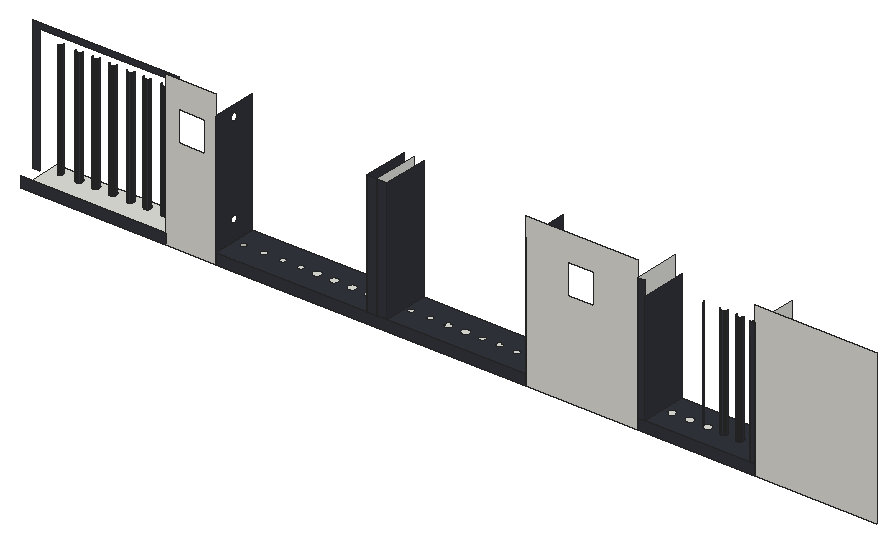
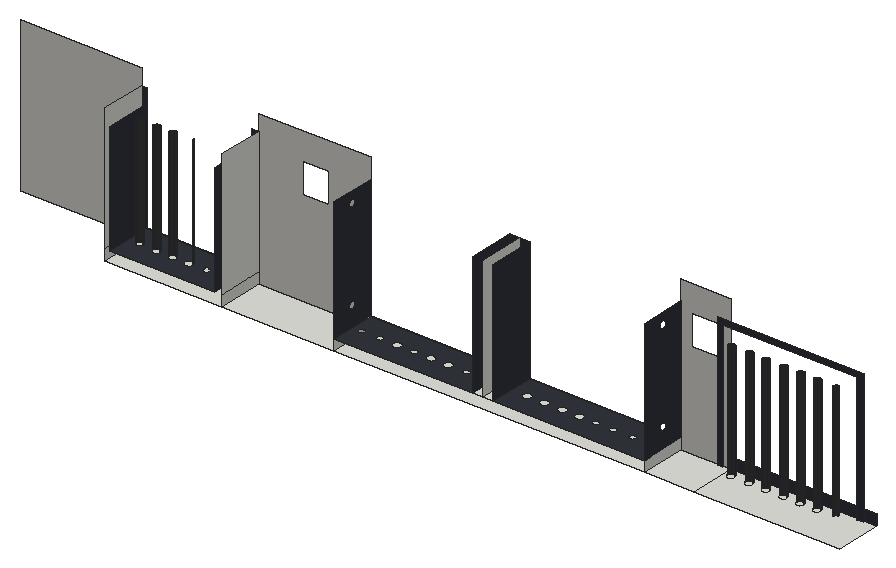
# SketchUp Ruby script. Lengths in inches.
U = 1.inch
M = Sketchup.active_model
def pt(a) = Geom::Point3d.new(a.map { |v| v * U })
def face(e, loops, mat)
  f = e.add_face(loops[0].map { |a| pt(a) })
  loops[1..].each { |l| e.add_face(l.map { |a| pt(a) }).erase! }
  f.material = f.back_material = mat if mat
  f
end
# faces: each face lists its corners as indices into pts; further lists are holes
def faces(e, pts, list, mat = nil) = list.each { |f| face(e, (f[0].is_a?(Array) ? f : [f]).map { |l| l.map { |i| pts[i] } }, mat) }
# xy, xz, yz: faces in a plane at the given z, y or x. An outline is a flat list of corners, or four numbers for a rectangle; further outlines are holes
def ring(l) = l.size == 4 ? [[l[0], l[1]], [l[2], l[1]], [l[2], l[3]], [l[0], l[3]]] : l.each_slice(2).to_a
def flat(e, list, mat, &to3) = list.each { |f| face(e, (f[0].is_a?(Array) ? f : [f]).map { |l| ring(l).map { |u, v| to3.(u, v) } }, mat) }
def xy(e, z, list, mat = nil) = flat(e, list, mat) { |x, y| [x, y, z] }
def xz(e, y, list, mat = nil) = flat(e, list, mat) { |x, z| [x, y, z] }
def yz(e, x, list, mat = nil) = flat(e, list, mat) { |y, z| [x, y, z] }
def lines(e, pts, list) = list.each { |a, b| e.add_line(pt(pts[a]), pt(pts[b])) }
# prism: a flat outline (further loops are holes) pulled along v
def prism(e, loops, v, mat = nil)
  f = face(e, loops, mat); d = Geom::Vector3d.new(v.map { |x| x * U })
  f.pushpull(f.normal.samedirection?(d) ? d.length : -d.length)
end
def box(e, o, s, mat = nil) = prism(e, [[o, [o[0] + s[0], o[1], o[2]], [o[0] + s[0], o[1] + s[1], o[2]], [o[0], o[1] + s[1], o[2]]]], [0, 0, s[2]], mat)
def at(x, y, z, deg = 0) = Geom::Transformation.translation(pt([x, y, z])) * Geom::Transformation.rotation(ORIGIN, Z_AXIS, deg.degrees)
def axes(o, x, y, z) = Geom::Transformation.new([*x, 0, *y, 0, *z, 0, *pt(o).to_a, 1])
def part(name) = M.definitions.add(name)
# library, detail: a bought-in or finely detailed component or shape, given as its bounding box
def library(name, o, s) = part(name).tap { |d| box(d.entities, o, s) }
def detail(e, o, s) = box(e.add_group.entities, o, s)
def put(e, d, t, mat = nil) = e.add_instance(d, t).tap { |i| i.material = mat if mat }
def group(e, t, mat = nil) = e.add_group.tap { |g| g.transformation = t; g.material = mat if mat }.entities
root = M.entities
M.materials.add("[Formica Laminate Dark]1").color = [50, 53, 60]
M.materials.add("[Terrazzo Tile Light]").color = [219, 217, 210]
xy(root,0,[[1357.59,0,1765.91,129.42],[1765.91,0,1905.75,129.42],[1905.75,0,2778.47,129.42],[2778.47,0,3092.67,129.42],[3092.67,0,3421.78,129.42]])
xy(root,29.875,[[2330.84,0,2358.7,129.42],[2358.7,0,2386.55,129.42],[1472.87,55.58,1470.36,55.72,1467.97,56.51,1465.87,57.89,1464.2,59.76,1463.07,62.01,1462.56,64.47,1462.7,66.98,1463.49,69.36,1464.86,71.46,1466.74,73.14,1468.98,74.27,1471.44,74.78,1473.95,74.64,1476.34,73.85,1478.4375,72.47,1480.11,70.6,1481.24,68.35,1481.75,65.89,1481.61,63.38,1480.82,61,1479.45,58.9,1477.57,57.22,1475.33,56.09],[1518.99,55.58,1516.48,55.72,1514.1,56.51,1512,57.89,1510.32,59.76,1509.19,62.01,1508.68,64.47,1508.82,66.98,1509.61,69.36,1510.99,71.46,1512.86,73.14,1515.11,74.27,1517.57,74.78,1520.08,74.64,1522.46,73.85,1524.5625,72.47,1526.24,70.6,1527.37,68.35,1527.88,65.89,1527.74,63.38,1526.95,61,1525.57,58.9,1523.7,57.22,1521.45,56.09],[1566.87,55.58,1564.36,55.72,1561.97,56.51,1559.87,57.89,1558.2,59.76,1557.07,62.01,1556.56,64.47,1556.7,66.98,1557.49,69.36,1558.86,71.46,1560.74,73.14,1562.98,74.27,1565.44,74.78,1567.95,74.64,1570.34,73.85,1572.4375,72.47,1574.11,70.6,1575.24,68.35,1575.75,65.89,1575.61,63.38,1574.82,61,1573.45,58.9,1571.57,57.22,1569.33,56.09],
  [1616.43,55.58,1613.92,55.72,1611.54,56.51,1609.43,57.89,1607.76,59.76,1606.63,62.01,1606.12,64.47,1606.26,66.98,1607.05,69.36,1608.43,71.46,1610.3,73.14,1612.54,74.27,1615,74.78,1617.51,74.64,1619.9,73.85,1622,72.47,1623.67,70.6,1624.8,68.35,1625.32,65.89,1625.17,63.38,1624.39,61,1623.01,58.9,1621.13,57.22,1618.89,56.09],[1663.87,55.58,1661.36,55.72,1658.97,56.51,1656.87,57.89,1655.2,59.76,1654.07,62.01,1653.56,64.47,1653.7,66.98,1654.49,69.36,1655.86,71.46,1657.74,73.14,1659.98,74.27,1662.44,74.78,1664.95,74.64,1667.34,73.85,1669.4375,72.47,1671.11,70.6,1672.24,68.35,1672.75,65.89,1672.61,63.38,1671.82,61,1670.45,58.9,1668.57,57.22,1666.33,56.09],[1714.37,55.58,1711.86,55.72,1709.47,56.51,1707.37,57.89,1705.7,59.76,1704.57,62.01,1704.06,64.47,1704.2,66.98,1704.99,69.36,1706.36,71.46,1708.24,73.14,1710.48,74.27,1712.94,74.78,1715.45,74.64,1717.84,73.85,1719.9375,72.47,1721.61,70.6,1722.74,68.35,1723.25,65.89,1723.11,63.38,1722.32,61,1720.95,58.9,1719.07,57.22,1716.83,56.09],[2139.99,55.58,2137.48,55.72,2135.1,56.51,2133,57.89,2131.32,59.76,2130.19,62.01,2129.68,64.47,2129.82,66.98,2130.61,69.36,2131.99,71.46,2133.86,73.14,2136.11,74.27,2138.57,74.78,2141.08,74.64,2143.46,73.85,2145.5625,72.47,2147.24,70.6,2148.37,68.35,2148.88,65.89,2148.74,63.38,2147.95,61,2146.57,58.9,2144.7,57.22,2142.45,56.09],[2187.99,55.58,2185.48,55.72,2183.1,56.51,2181,57.89,2179.32,59.76,2178.19,62.01,2177.68,64.47,2177.82,66.98,2178.61,69.36,2179.99,71.46,2181.86,73.14,2184.11,74.27,2186.57,74.78,2189.08,74.64,2191.46,73.85,2193.5625,72.47,2195.24,70.6,2196.37,68.35,2196.88,65.89,2196.74,63.38,2195.95,61,2194.57,58.9,2192.7,57.22,2190.45,56.09],
  [2238.68,55.58,2236.17,55.72,2233.79,56.51,2231.68,57.89,2230.01,59.76,2228.88,62.01,2228.37,64.47,2228.51,66.98,2229.3,69.36,2230.68,71.46,2232.55,73.14,2234.79,74.27,2237.25,74.78,2239.76,74.64,2242.15,73.85,2244.25,72.47,2245.92,70.6,2247.05,68.35,2247.57,65.89,2247.42,63.38,2246.64,61,2245.26,58.9,2243.38,57.22,2241.14,56.09],[2286.99,55.58,2284.48,55.72,2282.1,56.51,2280,57.89,2278.32,59.76,2277.19,62.01,2276.68,64.47,2276.82,66.98,2277.61,69.36,2278.99,71.46,2280.86,73.14,2283.11,74.27,2285.57,74.78,2288.08,74.64,2290.46,73.85,2292.5625,72.47,2294.24,70.6,2295.37,68.35,2295.88,65.89,2295.74,63.38,2294.95,61,2293.57,58.9,2291.7,57.22,2289.45,56.09],[2508.93,55.58,2506.42,55.72,2504.04,56.51,2501.93,57.89,2500.26,59.76,2499.13,62.01,2498.62,64.47,2498.76,66.98,2499.55,69.36,2500.93,71.46,2502.8,73.14,2505.04,74.27,2507.5,74.78,2510.01,74.64,2512.4,73.85,2514.5,72.47,2516.17,70.6,2517.3,68.35,2517.82,65.89,2517.67,63.38,2516.89,61,2515.51,58.9,2513.63,57.22,2511.39,56.09],[2557.49,55.58,2554.98,55.72,2552.6,56.51,2550.5,57.89,2548.82,59.76,2547.69,62.01,2547.18,64.47,2547.32,66.98,2548.11,69.36,2549.49,71.46,2551.36,73.14,2553.61,74.27,2556.07,74.78,2558.58,74.64,2560.96,73.85,2563.0625,72.47,2564.74,70.6,2565.87,68.35,2566.38,65.89,2566.24,63.38,2565.45,61,2564.07,58.9,2562.2,57.22,2559.95,56.09],[2651.93,55.58,2649.42,55.72,2647.04,56.51,2644.93,57.89,2643.26,59.76,2642.13,62.01,2641.62,64.47,2641.76,66.98,2642.55,69.36,2643.93,71.46,2645.8,73.14,2648.04,74.27,2650.5,74.78,2653.01,74.64,2655.4,73.85,2657.5,72.47,2659.17,70.6,2660.3,68.35,2660.82,65.89,2660.67,63.38,2659.89,61,2658.51,58.9,2656.63,57.22,2654.39,56.09],
  [3137.87,55.58,3135.36,55.72,3132.97,56.51,3130.87,57.89,3129.2,59.76,3128.07,62.01,3127.56,64.47,3127.7,66.98,3128.49,69.36,3129.86,71.46,3131.74,73.14,3133.98,74.27,3136.44,74.78,3138.95,74.64,3141.34,73.85,3143.4375,72.47,3145.11,70.6,3146.24,68.35,3146.75,65.89,3146.61,63.38,3145.82,61,3144.45,58.9,3142.57,57.22,3140.33,56.09],[3187.99,55.58,3185.48,55.72,3183.1,56.51,3181,57.89,3179.32,59.76,3178.19,62.01,3177.68,64.47,3177.82,66.98,3178.61,69.36,3179.99,71.46,3181.86,73.14,3184.11,74.27,3186.57,74.78,3189.08,74.64,3191.46,73.85,3193.5625,72.47,3195.24,70.6,3196.37,68.35,3196.88,65.89,3196.74,63.38,3195.95,61,3194.57,58.9,3192.7,57.22,3190.45,56.09],[3236.93,55.58,3234.42,55.72,3232.04,56.51,3229.93,57.89,3228.26,59.76,3227.13,62.01,3226.62,64.47,3226.76,66.98,3227.55,69.36,3228.93,71.46,3230.8,73.14,3233.04,74.27,3235.5,74.78,3238.01,74.64,3240.4,73.85,3242.5,72.47,3244.17,70.6,3245.3,68.35,3245.82,65.89,3245.67,63.38,3244.89,61,3243.51,58.9,3241.63,57.22,3239.39,56.09],[3282.55,55.58,3280.05,55.72,3277.66,56.51,3275.56,57.89,3273.89,59.76,3272.76,62.01,3272.24,64.47,3272.39,66.98,3273.17,69.36,3274.55,71.46,3276.43,73.14,3278.67,74.27,3281.13,74.78,3283.64,74.64,3286.02,73.85,3288.125,72.47,3289.8,70.6,3290.93,68.35,3291.44,65.89,3291.3,63.38,3290.51,61,3289.13,58.9,3287.26,57.22,3285.01,56.09],[3328.68,55.58,3326.17,55.72,3323.79,56.51,3321.68,57.89,3320.01,59.76,3318.88,62.01,3318.37,64.47,3318.51,66.98,3319.3,69.36,3320.68,71.46,3322.55,73.14,3324.79,74.27,3327.25,74.78,3329.76,74.64,3332.15,73.85,3334.25,72.47,3335.92,70.6,3337.05,68.35,3337.57,65.89,3337.42,63.38,3336.64,61,3335.26,58.9,3333.38,57.22,3331.14,56.09]])
xy(root,29.875,[[[1905.75,0,2330.84,129.42],[2139.99,55.58,2137.48,55.72,2135.1,56.51,2133,57.89,2131.32,59.76,2130.19,62.01,2129.68,64.47,2129.82,66.98,2130.61,69.36,2131.99,71.46,2133.86,73.14,2136.11,74.27,2138.57,74.78,2141.08,74.64,2143.46,73.85,2145.5625,72.47,2147.24,70.6,2148.37,68.35,2148.88,65.89,2148.74,63.38,2147.95,61,2146.57,58.9,2144.7,57.22,2142.45,56.09],[2187.99,55.58,2185.48,55.72,2183.1,56.51,2181,57.89,2179.32,59.76,2178.19,62.01,2177.68,64.47,2177.82,66.98,2178.61,69.36,2179.99,71.46,2181.86,73.14,2184.11,74.27,2186.57,74.78,2189.08,74.64,2191.46,73.85,2193.5625,72.47,2195.24,70.6,2196.37,68.35,2196.88,65.89,2196.74,63.38,2195.95,61,2194.57,58.9,2192.7,57.22,2190.45,56.09],[2238.68,55.58,2236.17,55.72,2233.79,56.51,2231.68,57.89,2230.01,59.76,2228.88,62.01,2228.37,64.47,2228.51,66.98,2229.3,69.36,2230.68,71.46,2232.55,73.14,2234.79,74.27,2237.25,74.78,2239.76,74.64,2242.15,73.85,2244.25,72.47,2245.92,70.6,2247.05,68.35,2247.57,65.89,2247.42,63.38,2246.64,61,2245.26,58.9,2243.38,57.22,2241.14,56.09],[2286.99,55.58,2284.48,55.72,2282.1,56.51,2280,57.89,2278.32,59.76,2277.19,62.01,2276.68,64.47,2276.82,66.98,2277.61,69.36,2278.99,71.46,2280.86,73.14,2283.11,74.27,2285.57,74.78,2288.08,74.64,2290.46,73.85,2292.5625,72.47,2294.24,70.6,2295.37,68.35,2295.88,65.89,2295.74,63.38,2294.95,61,2293.57,58.9,2291.7,57.22,2289.45,56.09],[2094.55,55.58,2092.05,55.72,2089.66,56.51,2087.56,57.89,2085.89,59.76,2084.76,62.01,2084.24,64.47,2084.39,66.98,2085.17,69.36,2086.55,71.46,2088.43,73.14,2090.67,74.27,2093.13,74.78,2095.64,74.64,2098.02,73.85,2100.125,72.47,2101.8,70.6,2102.93,68.35,2103.44,65.89,2103.3,63.38,2102.51,61,2101.13,58.9,2099.26,57.22,2097.01,56.09],[2044.37,55.58,2041.86,55.72,2039.47,56.51,2037.37,57.89,2035.7,59.76,2034.57,62.01,2034.06,64.47,2034.2,66.98,2034.99,69.36,2036.36,71.46,2038.24,73.14,2040.48,74.27,2042.94,74.78,2045.45,74.64,2047.84,73.85,2049.9375,72.47,2051.61,70.6,2052.74,68.35,2053.25,65.89,2053.11,63.38,2052.32,61,2050.95,58.9,2049.07,57.22,2046.83,56.09],[1934.18,55.58,1931.67,55.72,1929.29,56.51,1927.18,57.89,1925.51,59.76,1924.38,62.01,1923.87,64.47,1924.01,66.98,1924.8,69.36,1926.18,71.46,1928.05,73.14,1930.29,74.27,1932.75,74.78,1935.26,74.64,1937.65,73.85,1939.75,72.47,1941.42,70.6,1942.55,68.35,1943.07,65.89,1942.92,63.38,1942.14,61,1940.76,58.9,1938.88,57.22,1936.64,56.09],[1991.49,55.58,1988.98,55.72,1986.6,56.51,1984.5,57.89,1982.82,59.76,1981.69,62.01,1981.18,64.47,1981.32,66.98,1982.11,69.36,1983.49,71.46,1985.36,73.14,1987.61,74.27,1990.07,74.78,1992.58,74.64,1994.96,73.85,1997.0625,72.47,1998.74,70.6,1999.87,68.35,2000.38,65.89,2000.24,63.38,1999.45,61,1998.07,58.9,1996.2,57.22,1993.95,56.09]],[[2386.55,0,2778.47,129.42],[2508.93,55.58,2506.42,55.72,2504.04,56.51,2501.93,57.89,2500.26,59.76,2499.13,62.01,2498.62,64.47,2498.76,66.98,2499.55,69.36,2500.93,71.46,2502.8,73.14,2505.04,74.27,2507.5,74.78,2510.01,74.64,2512.4,73.85,2514.5,72.47,2516.17,70.6,2517.3,68.35,2517.82,65.89,2517.67,63.38,2516.89,61,2515.51,58.9,2513.63,57.22,2511.39,56.09],[2557.49,55.58,2554.98,55.72,2552.6,56.51,2550.5,57.89,2548.82,59.76,2547.69,62.01,2547.18,64.47,2547.32,66.98,2548.11,69.36,2549.49,71.46,2551.36,73.14,2553.61,74.27,2556.07,74.78,2558.58,74.64,2560.96,73.85,2563.0625,72.47,2564.74,70.6,2565.87,68.35,2566.38,65.89,2566.24,63.38,2565.45,61,2564.07,58.9,2562.2,57.22,2559.95,56.09],[2651.93,55.58,2649.42,55.72,2647.04,56.51,2644.93,57.89,2643.26,59.76,2642.13,62.01,2641.62,64.47,2641.76,66.98,2642.55,69.36,2643.93,71.46,2645.8,73.14,2648.04,74.27,2650.5,74.78,2653.01,74.64,2655.4,73.85,2657.5,72.47,2659.17,70.6,2660.3,68.35,2660.82,65.89,2660.67,63.38,2659.89,61,2658.51,58.9,2656.63,57.22,2654.39,56.09],[2752.12,55.58,2749.61,55.72,2747.22,56.51,2745.12,57.89,2743.45,59.76,2742.32,62.01,2741.81,64.47,2741.95,66.98,2742.74,69.36,2744.11,71.46,2745.99,73.14,2748.23,74.27,2750.69,74.78,2753.2,74.64,2755.59,73.85,2757.6875,72.47,2759.36,70.6,2760.49,68.35,2761,65.89,2760.86,63.38,2760.07,61,2758.7,58.9,2756.82,57.22,2754.58,56.09],[2700.93,55.58,2698.42,55.72,2696.04,56.51,2693.93,57.89,2692.26,59.76,2691.13,62.01,2690.62,64.47,2690.76,66.98,2691.55,69.36,2692.93,71.46,2694.8,73.14,2697.04,74.27,2699.5,74.78,2702.01,74.64,2704.4,73.85,2706.5,72.47,2708.17,70.6,2709.3,68.35,2709.82,65.89,2709.67,63.38,2708.89,61,2707.51,58.9,2705.63,57.22,2703.39,56.09],[2604.55,55.58,2602.05,55.72,2599.66,56.51,2597.56,57.89,2595.89,59.76,2594.76,62.01,2594.24,64.47,2594.39,66.98,2595.17,69.36,2596.55,71.46,2598.43,73.14,2600.67,74.27,2603.13,74.78,2605.64,74.64,2608.02,73.85,2610.125,72.47,2611.8,70.6,2612.93,68.35,2613.44,65.89,2613.3,63.38,2612.51,61,2611.13,58.9,2609.26,57.22,2607.01,56.09],[2458.12,55.58,2455.61,55.72,2453.22,56.51,2451.12,57.89,2449.45,59.76,2448.32,62.01,2447.81,64.47,2447.95,66.98,2448.74,69.36,2450.11,71.46,2451.99,73.14,2454.23,74.27,2456.69,74.78,2459.2,74.64,2461.59,73.85,2463.6875,72.47,2465.36,70.6,2466.49,68.35,2467,65.89,2466.86,63.38,2466.07,61,2464.7,58.9,2462.82,57.22,2460.58,56.09],[2404.12,55.58,2401.61,55.72,2399.22,56.51,2397.12,57.89,2395.45,59.76,2394.32,62.01,2393.81,64.47,2393.95,66.98,2394.74,69.36,2396.11,71.46,2397.99,73.14,2400.23,74.27,2402.69,74.78,2405.2,74.64,2407.59,73.85,2409.6875,72.47,2411.36,70.6,2412.49,68.35,2413,65.89,2412.86,63.38,2412.07,61,2410.7,58.9,2408.82,57.22,2406.58,56.09]],[[3111.49,0,3407.39,129.42],[3328.68,55.58,3326.17,55.72,3323.79,56.51,3321.68,57.89,3320.01,59.76,3318.88,62.01,3318.37,64.47,3318.51,66.98,3319.3,69.36,3320.68,71.46,3322.55,73.14,3324.79,74.27,3327.25,74.78,3329.76,74.64,3332.15,73.85,3334.25,72.47,3335.92,70.6,3337.05,68.35,3337.57,65.89,3337.42,63.38,3336.64,61,3335.26,58.9,3333.38,57.22,3331.14,56.09],[3137.87,55.58,3135.36,55.72,3132.97,56.51,3130.87,57.89,3129.2,59.76,3128.07,62.01,3127.56,64.47,3127.7,66.98,3128.49,69.36,3129.86,71.46,3131.74,73.14,3133.98,74.27,3136.44,74.78,3138.95,74.64,3141.34,73.85,3143.4375,72.47,3145.11,70.6,3146.24,68.35,3146.75,65.89,3146.61,63.38,3145.82,61,3144.45,58.9,3142.57,57.22,3140.33,56.09],[3282.55,55.58,3280.05,55.72,3277.66,56.51,3275.56,57.89,3273.89,59.76,3272.76,62.01,3272.24,64.47,3272.39,66.98,3273.17,69.36,3274.55,71.46,3276.43,73.14,3278.67,74.27,3281.13,74.78,3283.64,74.64,3286.02,73.85,3288.125,72.47,3289.8,70.6,3290.93,68.35,3291.44,65.89,3291.3,63.38,3290.51,61,3289.13,58.9,3287.26,57.22,3285.01,56.09],[3187.99,55.58,3185.48,55.72,3183.1,56.51,3181,57.89,3179.32,59.76,3178.19,62.01,3177.68,64.47,3177.82,66.98,3178.61,69.36,3179.99,71.46,3181.86,73.14,3184.11,74.27,3186.57,74.78,3189.08,74.64,3191.46,73.85,3193.5625,72.47,3195.24,70.6,3196.37,68.35,3196.88,65.89,3196.74,63.38,3195.95,61,3194.57,58.9,3192.7,57.22,3190.45,56.09],[3236.93,55.58,3234.42,55.72,3232.04,56.51,3229.93,57.89,3228.26,59.76,3227.13,62.01,3226.62,64.47,3226.76,66.98,3227.55,69.36,3228.93,71.46,3230.8,73.14,3233.04,74.27,3235.5,74.78,3238.01,74.64,3240.4,73.85,3242.5,72.47,3244.17,70.6,3245.3,68.35,3245.82,65.89,3245.67,63.38,3244.89,61,3243.51,58.9,3241.63,57.22,3239.39,56.09],[3376.3,55.58,3373.8,55.72,3371.41,56.51,3369.31,57.89,3367.64,59.76,3366.51,62.01,3365.99,64.47,3366.14,66.98,3366.92,69.36,3368.3,71.46,3370.18,73.14,3372.42,74.27,3374.88,74.78,3377.39,74.64,3379.77,73.85,3381.875,72.47,3383.55,70.6,3384.68,68.35,3385.19,65.89,3385.05,63.38,3384.26,61,3382.88,58.9,3381.01,57.22,3378.76,56.09]]],"[Formica Laminate Dark]1")
xz(root,0,[[1357.59,0,1765.91,29.875],[1905.75,0,2778.47,29.875],[3092.67,0,3421.78,29.875],[2330.84,29.875,2358.7,373.47],[2358.7,29.875,2386.55,373.47],
  [3092.67,29.875,3111.49,384.04],[3407.39,29.875,3421.78,384.04]],"[Formica Laminate Dark]1")
xz(root,0,[[[1765.91,0,1905.75,429.3125],[1802.64,268.73,1875.77,354.42]],[[2778.47,0,3092.67,429.3125],[2895.58,268.73,2968.71,354.42]],[3421.78,0,3762.625,429.3125]],"[Terrazzo Tile Light]")
xz(root,44.85,[[1357.59,29.875,1376.86,29.875,1376.86,387.92,1752.89,387.92,1752.89,29.875,1765.91,29.875,1765.91,402.23,1357.59,402.23]],"[Formica Laminate Dark]1")
yz(root,1905.75,[[0,0,129.42,29.875]])
yz(root,1905.75,[[[0,29.875,129.42,373.47],[64.71,332.24,61.98,332.6,59.43,333.66,57.24,335.33,55.5625,337.52,54.51,340.07,54.15,342.8,54.51,345.54,55.5625,348.08,57.24,350.27,59.43,351.95,61.98,353.01,64.71,353.37,67.44,353.01,69.99,351.95,72.18,350.27,73.86,348.08,74.91,345.54,75.27,342.8,74.91,340.07,73.86,337.52,72.18,335.33,69.99,333.66,67.44,332.6],[64.71,75.12,61.98,75.48,59.43,76.53,57.24,78.21,55.5625,80.4,54.51,82.94,54.15,85.68,54.51,88.41,55.5625,90.96,57.24,93.15,59.43,94.83,61.98,95.88,64.71,96.24,67.44,95.88,69.99,94.83,72.18,93.15,73.86,90.96,74.91,88.41,75.27,85.68,74.91,82.94,73.86,80.4,72.18,78.21,69.99,76.53,67.44,75.48]]],"[Formica Laminate Dark]1")
yz(root,2330.84,[[0,29.875,129.42,373.47]],"[Formica Laminate Dark]1")
yz(root,2358.7,[[0,29.875,129.42,373.47]])
yz(root,2386.55,[[0,29.875,129.42,373.47]],"[Formica Laminate Dark]1")
yz(root,2778.47,[[0,0,129.42,29.875]])
yz(root,2778.47,[[[0,29.875,129.42,373.47],[64.71,332.24,67.44,332.6,69.99,333.66,72.18,335.33,73.86,337.52,74.91,340.07,75.27,342.8,74.91,345.54,73.86,348.08,72.18,350.27,69.99,351.95,67.44,353.01,64.71,353.37,61.98,353.01,59.43,351.95,57.24,350.27,55.5625,348.08,54.51,345.54,54.15,342.8,54.51,340.07,55.5625,337.52,57.24,335.33,59.43,333.66,61.98,332.6],[64.71,75.12,67.44,75.48,69.99,76.53,72.18,78.21,73.86,80.4,74.91,82.94,75.27,85.68,74.91,88.41,73.86,90.96,72.18,93.15,69.99,94.83,67.44,95.88,64.71,96.24,61.98,95.88,59.43,94.83,57.24,93.15,55.5625,90.96,54.51,88.41,54.15,85.68,54.51,82.94,55.5625,80.4,57.24,78.21,59.43,76.53,61.98,75.48]]],"[Formica Laminate Dark]1")
yz(root,3092.67,[[0,0,129.42,29.875],[0,29.875,129.42,384.04]])
yz(root,3111.49,[[0,29.875,129.42,342.54]],"[Formica Laminate Dark]1")
yz(root,3407.39,[[0,29.875,129.42,342.54]],"[Formica Laminate Dark]1")
yz(root,3421.78,[[0,0,129.42,29.875],[0,29.875,129.42,384.04]])
p = [[1417.24,55.58,29.875],[1419.7,56.09,29.875],[1419.7,56.09,357.02],[1417.24,55.58,357.02],[1470.36,55.72,29.875],[1472.87,55.58,29.875],
  [1472.87,55.58,357.02],[1470.36,55.72,357.02],[1475.33,56.09,29.875],[1475.33,56.09,357.02],[1516.48,55.72,29.875],[1518.99,55.58,29.875],
  [1518.99,55.58,357.02],[1516.48,55.72,357.02],[1521.45,56.09,29.875],[1521.45,56.09,357.02],[1564.36,55.72,29.875],[1566.87,55.58,29.875],
  [1566.87,55.58,357.02],[1564.36,55.72,357.02],[1569.33,56.09,29.875],[1569.33,56.09,357.02],[1613.92,55.72,29.875],[1616.43,55.58,29.875],
  [1616.43,55.58,357.02],[1613.92,55.72,357.02],[1618.89,56.09,29.875],[1618.89,56.09,357.02],[1661.36,55.72,29.875],[1663.87,55.58,29.875],
  [1663.87,55.58,357.02],[1661.36,55.72,357.02],[1666.33,56.09,29.875],[1666.33,56.09,357.02],[1711.86,55.72,29.875],[1714.37,55.58,29.875],
  [1714.37,55.58,357.02],[1711.86,55.72,357.02],[1716.83,56.09,29.875],[1716.83,56.09,357.02],[3280.05,55.72,29.875],[3282.55,55.58,29.875],
  [3282.55,55.58,342.54],[3280.05,55.72,342.54],[3285.01,56.09,29.875],[3285.01,56.09,342.54],[3326.17,55.72,29.875],[3328.68,55.58,29.875],
  [3328.68,55.58,342.54],[3326.17,55.72,342.54],[3331.14,56.09,29.875],[3331.14,56.09,342.54],[3373.8,55.72,29.875],[3376.3,55.58,29.875],
  [3376.3,55.58,342.54],[3373.8,55.72,342.54],[3378.76,56.09,29.875],[3378.76,56.09,342.54],[1467.97,56.51,29.875],[1467.97,56.51,357.02],
  [1514.1,56.51,29.875],[1514.1,56.51,357.02],[1561.97,56.51,29.875],[1561.97,56.51,357.02],[1611.54,56.51,29.875],[1611.54,56.51,357.02],
  [1658.97,56.51,29.875],[1658.97,56.51,357.02],[1709.47,56.51,29.875],[1709.47,56.51,357.02],[3277.66,56.51,29.875],[3277.66,56.51,342.54],
  [3323.79,56.51,29.875],[3323.79,56.51,342.54],[3371.41,56.51,29.875],[3371.41,56.51,342.54],[1421.95,57.22,29.875],[1421.95,57.22,357.02],
  [1477.57,57.22,29.875],[1477.57,57.22,357.02],[1523.7,57.22,29.875],[1523.7,57.22,357.02],[1571.57,57.22,29.875],[1571.57,57.22,357.02],
  [1621.13,57.22,29.875],[1621.13,57.22,357.02],[1668.57,57.22,29.875],[1668.57,57.22,357.02],[1719.07,57.22,29.875],[1719.07,57.22,357.02],
  [3287.26,57.22,29.875],[3287.26,57.22,342.54],[3333.38,57.22,29.875],[3333.38,57.22,342.54],[3381.01,57.22,29.875],[3381.01,57.22,342.54],
  [1465.87,57.89,29.875],[1465.87,57.89,357.02],[1512,57.89,29.875],[1512,57.89,357.02],[1559.87,57.89,29.875],[1559.87,57.89,357.02],
  [1609.43,57.89,29.875],[1609.43,57.89,357.02],[1656.87,57.89,29.875],[1656.87,57.89,357.02],[1707.37,57.89,29.875],[1707.37,57.89,357.02],
  [3275.56,57.89,29.875],[3275.56,57.89,342.54],[3321.68,57.89,29.875],[3321.68,57.89,342.54],[3369.31,57.89,29.875],[3369.31,57.89,342.54],
  [1423.82,58.9,29.875],[1423.82,58.9,357.02],[1479.45,58.9,29.875],[1479.45,58.9,357.02],[1525.57,58.9,29.875],[1525.57,58.9,357.02],
  [1573.45,58.9,29.875],[1573.45,58.9,357.02],[1623.01,58.9,29.875],[1623.01,58.9,357.02],[1670.45,58.9,29.875],[1670.45,58.9,357.02],
  [1720.95,58.9,29.875],[1720.95,58.9,357.02],[3289.13,58.9,29.875],[3289.13,58.9,342.54],[3335.26,58.9,29.875],[3335.26,58.9,342.54],
  [3382.88,58.9,29.875],[3382.88,58.9,342.54],[1464.2,59.76,29.875],[1464.2,59.76,357.02],[1510.32,59.76,29.875],[1510.32,59.76,357.02],
  [1558.2,59.76,29.875],[1558.2,59.76,357.02],[1607.76,59.76,29.875],[1607.76,59.76,357.02],[1655.2,59.76,29.875],[1655.2,59.76,357.02],
  [1705.7,59.76,29.875],[1705.7,59.76,357.02],[3228.26,59.76,29.875],[3229.93,57.89,29.875],[3229.93,57.89,342.54],[3228.26,59.76,342.54],
  [3273.89,59.76,29.875],[3273.89,59.76,342.54],[3320.01,59.76,29.875],[3320.01,59.76,342.54],[3367.64,59.76,29.875],[3367.64,59.76,342.54],
  [1425.2,61,29.875],[1425.2,61,357.02],[1480.82,61,29.875],[1480.82,61,357.02],[1526.95,61,29.875],[1526.95,61,357.02],
  [1574.82,61,29.875],[1574.82,61,357.02],[1624.39,61,29.875],[1624.39,61,357.02],[1671.82,61,29.875],[1671.82,61,357.02],
  [1722.32,61,29.875],[1722.32,61,357.02],[3290.51,61,29.875],[3290.51,61,342.54],[3336.64,61,29.875],[3336.64,61,342.54],
  [3384.26,61,29.875],[3384.26,61,342.54],[1463.07,62.01,29.875],[1463.07,62.01,357.02],[1509.19,62.01,29.875],[1509.19,62.01,357.02],
  [1557.07,62.01,29.875],[1557.07,62.01,357.02],[1606.63,62.01,29.875],[1606.63,62.01,357.02],[1654.07,62.01,29.875],[1654.07,62.01,357.02],
  [1704.57,62.01,29.875],[1704.57,62.01,357.02],[3227.13,62.01,29.875],[3227.13,62.01,342.54],[3272.76,62.01,29.875],[3272.76,62.01,342.54],
  [3318.88,62.01,29.875],[3318.88,62.01,342.54],[3366.51,62.01,29.875],[3366.51,62.01,342.54],[1425.99,63.38,29.875],[1425.99,63.38,357.02],
  [1481.61,63.38,29.875],[1481.61,63.38,357.02],[1527.74,63.38,29.875],[1527.74,63.38,357.02],[1575.61,63.38,29.875],[1575.61,63.38,357.02],
  [1625.17,63.38,29.875],[1625.17,63.38,357.02],[1672.61,63.38,29.875],[1672.61,63.38,357.02],[1723.11,63.38,29.875],[1723.11,63.38,357.02],
  [3291.3,63.38,29.875],[3291.3,63.38,342.54],[3337.42,63.38,29.875],[3337.42,63.38,342.54],[3385.05,63.38,29.875],[3385.05,63.38,342.54],
  [1462.56,64.47,29.875],[1462.56,64.47,357.02],[1508.68,64.47,29.875],[1508.68,64.47,357.02],[1556.56,64.47,29.875],[1556.56,64.47,357.02],
  [1606.12,64.47,29.875],[1606.12,64.47,357.02],[1653.56,64.47,29.875],[1653.56,64.47,357.02],[1704.06,64.47,29.875],[1704.06,64.47,357.02],
  [3226.62,64.47,29.875],[3226.62,64.47,342.54],[3272.24,64.47,29.875],[3272.24,64.47,342.54],[3318.37,64.47,29.875],[3318.37,64.47,342.54],
  [3365.99,64.47,29.875],[3365.99,64.47,342.54],[1426.13,65.89,29.875],[1426.13,65.89,357.02],[1481.75,65.89,29.875],[1481.75,65.89,357.02],
  [1527.88,65.89,29.875],[1527.88,65.89,357.02],[1575.75,65.89,29.875],[1575.75,65.89,357.02],[1625.32,65.89,29.875],[1625.32,65.89,357.02],
  [1672.75,65.89,29.875],[1672.75,65.89,357.02],[1723.25,65.89,29.875],[1723.25,65.89,357.02],[3291.44,65.89,29.875],[3291.44,65.89,342.54],
  [3337.57,65.89,29.875],[3337.57,65.89,342.54],[3385.19,65.89,29.875],[3385.19,65.89,342.54]]
faces(root,p,[[0,1,2,3],[4,5,6,7],[5,8,9,6],[10,11,12,13],[11,14,15,12],[16,17,18,19],[17,20,21,18],[22,23,24,25],
  [23,26,27,24],[28,29,30,31],[29,32,33,30],[34,35,36,37],[35,38,39,36],[40,41,42,43],[41,44,45,42],[46,47,48,49],
  [47,50,51,48],[52,53,54,55],[53,56,57,54],[58,4,7,59],[60,10,13,61],[62,16,19,63],[64,22,25,65],[66,28,31,67],
  [68,34,37,69],[70,40,43,71],[72,46,49,73],[74,52,55,75],[1,76,77,2],[8,78,79,9],[14,80,81,15],[20,82,83,21],
  [26,84,85,27],[32,86,87,33],[38,88,89,39],[44,90,91,45],[50,92,93,51],[56,94,95,57],[96,58,59,97],[98,60,61,99],
  [100,62,63,101],[102,64,65,103],[104,66,67,105],[106,68,69,107],[108,70,71,109],[110,72,73,111],[112,74,75,113],[76,114,115,77],
  [78,116,117,79],[80,118,119,81],[82,120,121,83],[84,122,123,85],[86,124,125,87],[88,126,127,89],[90,128,129,91],[92,130,131,93],
  [94,132,133,95],[134,96,97,135],[136,98,99,137],[138,100,101,139],[140,102,103,141],[142,104,105,143],[144,106,107,145],[146,147,148,149],
  [150,108,109,151],[152,110,111,153],[154,112,113,155],[114,156,157,115],[116,158,159,117],[118,160,161,119],[120,162,163,121],[122,164,165,123],
  [124,166,167,125],[126,168,169,127],[128,170,171,129],[130,172,173,131],[132,174,175,133],[176,134,135,177],[178,136,137,179],[180,138,139,181],
  [182,140,141,183],[184,142,143,185],[186,144,145,187],[188,146,149,189],[190,150,151,191],[192,152,153,193],[194,154,155,195],[156,196,197,157],
  [158,198,199,159],[160,200,201,161],[162,202,203,163],[164,204,205,165],[166,206,207,167],[168,208,209,169],[170,210,211,171],[172,212,213,173],
  [174,214,215,175],[216,176,177,217],[218,178,179,219],[220,180,181,221],[222,182,183,223],[224,184,185,225],[226,186,187,227],[228,188,189,229],
  [230,190,191,231],[232,192,193,233],[234,194,195,235],[196,236,237,197],[198,238,239,199],[200,240,241,201],[202,242,243,203],[204,244,245,205],
  [206,246,247,207],[208,248,249,209],[210,250,251,211],[212,252,253,213],[214,254,255,215]],"[Formica Laminate Dark]1")
